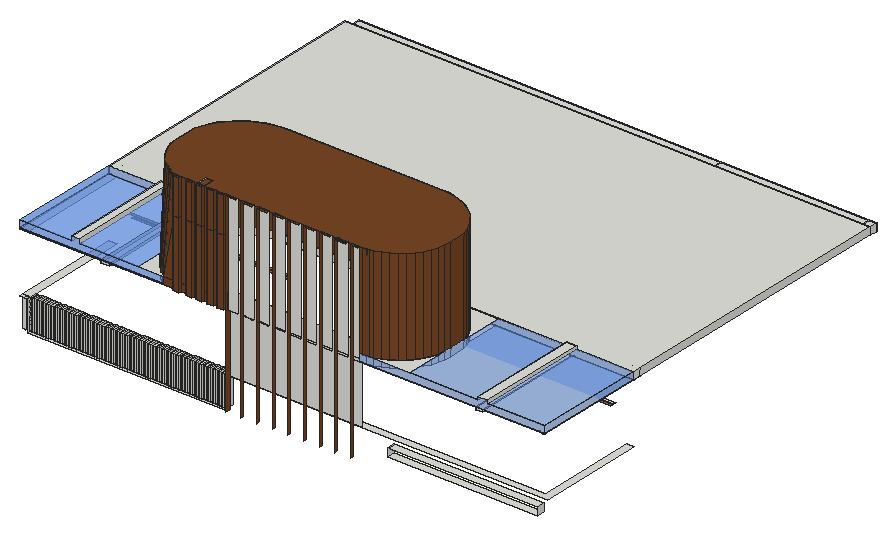
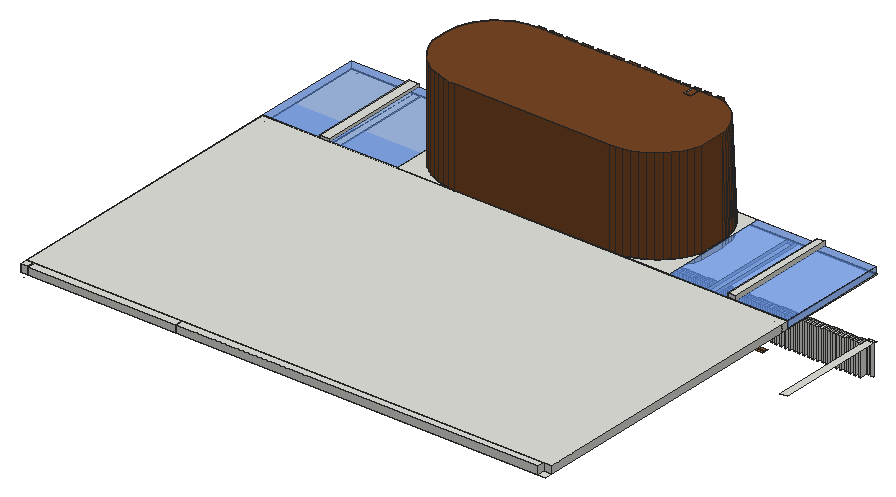
# SketchUp Ruby script. Lengths in inches.
U = 1.inch
M = Sketchup.active_model
def pt(a) = Geom::Point3d.new(a.map { |v| v * U })
def face(e, loops, mat)
  f = e.add_face(loops[0].map { |a| pt(a) })
  loops[1..].each { |l| e.add_face(l.map { |a| pt(a) }).erase! }
  f.material = f.back_material = mat if mat
  f
end
# faces: each face lists its corners as indices into pts; further lists are holes
def faces(e, pts, list, mat = nil) = list.each { |f| face(e, (f[0].is_a?(Array) ? f : [f]).map { |l| l.map { |i| pts[i] } }, mat) }
# xy, xz, yz: faces in a plane at the given z, y or x. An outline is a flat list of corners, or four numbers for a rectangle; further outlines are holes
def ring(l) = l.size == 4 ? [[l[0], l[1]], [l[2], l[1]], [l[2], l[3]], [l[0], l[3]]] : l.each_slice(2).to_a
def flat(e, list, mat, &to3) = list.each { |f| face(e, (f[0].is_a?(Array) ? f : [f]).map { |l| ring(l).map { |u, v| to3.(u, v) } }, mat) }
def xy(e, z, list, mat = nil) = flat(e, list, mat) { |x, y| [x, y, z] }
def xz(e, y, list, mat = nil) = flat(e, list, mat) { |x, z| [x, y, z] }
def yz(e, x, list, mat = nil) = flat(e, list, mat) { |y, z| [x, y, z] }
def lines(e, pts, list) = list.each { |a, b| e.add_line(pt(pts[a]), pt(pts[b])) }
# prism: a flat outline (further loops are holes) pulled along v
def prism(e, loops, v, mat = nil)
  f = face(e, loops, mat); d = Geom::Vector3d.new(v.map { |x| x * U })
  f.pushpull(f.normal.samedirection?(d) ? d.length : -d.length)
end
def box(e, o, s, mat = nil) = prism(e, [[o, [o[0] + s[0], o[1], o[2]], [o[0] + s[0], o[1] + s[1], o[2]], [o[0], o[1] + s[1], o[2]]]], [0, 0, s[2]], mat)
def at(x, y, z, deg = 0) = Geom::Transformation.translation(pt([x, y, z])) * Geom::Transformation.rotation(ORIGIN, Z_AXIS, deg.degrees)
def axes(o, x, y, z) = Geom::Transformation.new([*x, 0, *y, 0, *z, 0, *pt(o).to_a, 1])
def part(name) = M.definitions.add(name)
# library, detail: a bought-in or finely detailed component or shape, given as its bounding box
def library(name, o, s) = part(name).tap { |d| box(d.entities, o, s) }
def detail(e, o, s) = box(e.add_group.entities, o, s)
def put(e, d, t, mat = nil) = e.add_instance(d, t).tap { |i| i.material = mat if mat }
def group(e, t, mat = nil) = e.add_group.tap { |g| g.transformation = t; g.material = mat if mat }.entities
root = M.entities
M.materials.add("[Translucent Glass Blue]").color = [100, 149, 237]
M.materials["[Translucent Glass Blue]"].alpha = 0.5
M.materials.add("[Wood Bamboo]").color = [177, 105, 43]
M.materials.add("[Wood Veneer 01]").color = [120, 70, 37]
xy(root,503.6,[[9.45,3,248.625,6],[9.45,6,11.73,15],[15,6,17.29,15],[20.5625,6,22.86,15],[26.125,6,28.42,15],
  [31.6875,6,33.98,15],[37.25,6,39.54,15],[42.8125,6,45.11,15],[48.375,6,50.67,15],[53.9375,6,56.23,15],
  [59.5,6,61.79,15],[65.0625,6,67.36,15],[70.625,6,72.92,15],[76.1875,6,78.48,15],[81.75,6,84.04,15],
  [87.3125,6,89.61,15],[92.875,6,95.17,15],[98.4375,6,100.73,15],[104,6,106.29,15],[109.5625,6,111.86,15],
  [115.125,6,117.42,15],[120.6875,6,122.98,15],[126.25,6,128.54,15],[131.8125,6,134.11,15],[137.375,6,139.67,15],
  [142.9375,6,145.23,15],[148.5,6,150.79,15],[154.0625,6,156.36,15],[159.625,6,161.92,15],[165.1875,6,167.48,15],
  [170.75,6,173.04,15],[176.3125,6,178.61,15],[181.875,6,184.17,15],[187.4375,6,189.73,15],[193,6,195.29,15],
  [198.5625,6,200.86,15],[204.125,6,206.42,15],[209.6875,6,211.98,15],[215.25,6,217.54,15],[220.8125,6,223.11,15],
  [226.375,6,228.67,15],[231.9375,6,234.23,15],[237.5,6,239.79,15],[243.0625,6,245.36,15]])
xy(root,519.5625,[[439.02,6,618.46,15]])
xy(root,529,[[439.02,6,618.46,15]])
xy(root,540,[[0,3,9.45,6],[0,6,9.45,6,9.45,15,9,15,9,136.3125,0,136.3125],[11.73,6,15,15],[17.29,6,20.5625,15],[22.86,6,26.125,15],
  [28.42,6,31.6875,15],[33.98,6,37.25,15],[39.54,6,42.8125,15],[45.11,6,48.375,15],[50.67,6,53.9375,15],
  [56.23,6,59.5,15],[61.79,6,65.0625,15],[67.36,6,70.625,15],[72.92,6,76.1875,15],[78.48,6,81.75,15],
  [84.04,6,87.3125,15],[89.61,6,92.875,15],[95.17,6,98.4375,15],[100.73,6,104,15],[106.29,6,109.5625,15],
  [111.86,6,115.125,15],[117.42,6,120.6875,15],[122.98,6,126.25,15],[128.54,6,131.8125,15],[134.11,6,137.375,15],
  [139.67,6,142.9375,15],[145.23,6,148.5,15],[150.79,6,154.0625,15],[156.36,6,159.625,15],[161.92,6,165.1875,15],
  [167.48,6,170.75,15],[173.04,6,176.3125,15],[178.61,6,181.875,15],[184.17,6,187.4375,15],[189.73,6,193,15],
  [195.29,6,198.5625,15],[200.86,6,204.125,15],[206.42,6,209.6875,15],[211.98,6,215.25,15],[217.54,6,220.8125,15],
  [223.11,6,226.375,15],[228.67,6,231.9375,15],[234.23,6,237.5,15],[239.79,6,243.0625,15],[245.36,6,630,6,630,136.3125,621,136.3125,621,15,245.36,15]])
xy(root,576.5625,[[29.31,133.3125,65.31,136.3125],[69.34,133.3125,101.31,136.3125],[143.85,133.3125,179.85,136.3125],[182.97,133.3125,215.85,136.3125],[428.86,133.3125,464.86,136.3125],
  [469.18,133.3125,500.86,136.3125],[532.86,133.3125,568.86,136.3125],[572.23,133.3125,604.86,136.3125]],"[Wood Bamboo]")
xy(root,579.5625,[[425.86,133.3125,503.86,136.3125],[529.86,133.3125,607.86,136.3125]])
xy(root,579.5625,[[26.31,133.3125,104.31,136.3125],[140.85,133.3125,218.85,136.3125]],"[Wood Bamboo]")
xy(root,612,[[185.21,0,193.08,3],[200.4,0,208.27,3],[212.61,0,220.48,3],[226.11,0,233.98,3],[238.11,0,245.98,3],
  [0,3,9,136.3125],[0,136.3125,9,145.3125],[9,136.3125,629.5625,145.3125],[629.5625,136.3125,630,136.94],[629.5625,136.94,630,145.3125],
  [0,145.3125,9,490.375],[9,145.3125,621,490.375],[621,145.3125,629.5625,490.375],[629.5625,145.3125,630,490.375],[0,490.375,9,499.375],
  [9,490.375,443.23,499.375],[443.23,490.375,620.5,499.375],[620.5,490.375,620.75,497.0625],[620.75,490.375,621,499.375],[621,490.375,628.8125,499.375],
  [628.8125,490.375,629.5625,499.375],[629.5625,490.375,630,499.375],[620.5,497.0625,620.75,499.3125],[620.5,499.3125,620.75,499.375]])
xy(root,612.0625,[[406.875,3,414.84,3.52,422.66,5.08,430.22,7.64,437.375,11.17,444.01,15.6,450.01,20.87,455.27,26.86,459.7,33.5,463.23,40.65,465.79,48.21,467.35,56.03,467.87,64,467.87,83.88,465.38,91.23,462.12,98.27,458.11,104.91,453.41,111.08,448.07,116.7,442.15,121.72,435.73,126.07,428.87,129.7,421.66,132.57,414.1875,134.64,406.53,135.89,398.79,136.3125,629.5625,136.3125,629.5625,3]])
xy(root,612.75,[[0,3,0,136.3125,213.71,136.3125,205.95,135.9,198.27,134.65,190.78,132.6,183.55,129.75,176.66,126.15,170.2,121.83,164.24,116.84,158.84,111.25,154.08,105.11,149.99,98.5,146.64,91.48,144.06,84.15,144.06,52.64,144.28,47.64,144.93,42.68,146.01,37.8,147.51,33.03,149.43,28.41,151.73,23.98,154.42,19.76,157.46,15.8,160.84,12.11,164.53,8.73,168.49,5.6875,172.71,3]],"[Translucent Glass Blue]")
xy(root,621,[[142.34,3,172.71,3,168.49,5.6875,164.53,8.73,160.84,12.11,157.46,15.8,154.42,19.76,151.73,23.98,149.43,28.41,147.51,33.03,146.01,37.8,144.93,42.68,144.28,47.64,144.06,52.64,144.06,84.15,146.64,91.48,149.99,98.5,154.08,105.11,158.84,111.25,164.24,116.84,170.2,121.83,176.66,126.15,183.55,129.75,190.78,132.6,198.27,134.65,205.95,135.9,213.71,136.3125,142.34,136.3125],[406.875,3,467.9,3,467.9,136.3125,398.79,136.3125,406.53,135.89,414.1875,134.64,421.66,132.57,428.87,129.7,435.73,126.07,442.15,121.72,448.07,116.7,453.41,111.08,458.11,104.91,462.12,98.27,465.38,91.23,467.87,83.88,467.87,64,467.35,56.03,465.79,48.21,463.23,40.65,459.7,33.5,455.27,26.86,450.01,20.87,444.01,15.6,437.375,11.17,430.22,7.64,422.66,5.08,414.84,3.52],[0,136.3125,630,490.375],[9,490.375,443.23,499.375],[443.23,490.375,620.5,499.375],
  [621,490.375,630,499.375]])
xy(root,621,[[0,3,62.18,136.3125],[71.17,3,142.34,136.3125],[467.9,3,548.73,136.3125],[560.78,3,629.5625,136.3125]],"[Translucent Glass Blue]")
xy(root,624.3125,[[548.73,3,560.78,136.3125]])
xy(root,626.25,[[62.18,3,71.17,136.3125]])
xy(root,692.5,[[185.21,0,193.08,3],[200.4,0,208.27,3],[212.61,0,220.48,3],[226.11,0,233.98,3],[238.11,0,245.98,3],
  [212.61,3,220.48,15.6875]])
xy(root,735.21,[[380.31,0,392.78,3]])
xy(root,735.4375,[[185.21,0,193.08,3],[200.4,0,208.27,3],[212.61,0,220.48,3],[226.11,0,233.98,3],[238.11,0,245.98,3],
  [248.625,0,261.1,3],[267.4375,0,279.91,3],[286.25,0,298.72,3],[305.06,0,317.53,3],[323.87,0,336.34,3],
  [342.68,0,355.16,3],[361.49,0,373.97,3],[380.31,0,392.78,3],[399.12,0,406.875,3],[185.21,3,212.61,3,212.61,15.6875,220.48,15.6875,220.48,3,406.875,3,410.86,3.26,414.84,3.52,422.66,5.08,430.22,7.64,437.375,11.17,444.01,15.6,450.01,20.87,455.27,26.86,459.7,33.5,463.23,40.65,465.79,48.21,467.35,56.03,467.87,64,467.87,83.88,465.38,91.23,462.12,98.27,458.11,104.91,453.41,111.08,448.07,116.7,442.15,121.72,435.73,126.07,428.87,129.7,421.66,132.57,414.1875,134.64,406.53,135.89,398.79,136.3125,213.71,136.3125,205.95,135.9,198.27,134.65,190.78,132.6,183.55,129.75,176.66,126.15,170.2,121.83,164.24,116.84,158.84,111.25,154.08,105.11,149.99,98.5,146.64,91.48,144.06,84.15,144.06,52.64,145.24,47.14,146.9,41.76,149.02,36.55,151.59,31.55,154.59,26.79,157.98,22.31,161.76,18.14,165.88,14.3125,170.33,10.86,175.05,7.81,180.03,5.18],
  [212.61,3,220.48,15.6875]],"[Wood Veneer 01]")
xz(root,0,[[185.21,612,193.08,692.5],[200.4,612,208.27,692.5],[212.61,612,220.48,692.5],[226.11,612,233.98,692.5],[238.11,612,245.98,692.5],
  [185.21,692.5,193.08,735.4375],[200.4,692.5,208.27,735.4375],[212.61,692.5,220.48,735.4375],[226.11,692.5,233.98,735.4375],[238.11,692.5,245.98,735.4375],
  [380.31,735.21,392.78,735.4375]],"[Wood Veneer 01]")
xz(root,3,[[546.58,609.5,555.5,609.5,555.5,612,629.5625,612,629.5625,612.0625,406.875,612.0625,406.875,612,546.58,612],[185.21,612,193.08,621],[200.4,612,208.27,621],[212.61,612,220.48,621],[226.11,612,233.98,621],
  [238.11,612,245.98,621],[248.625,612,261.1,735.4375],[267.4375,612,279.91,612.375],[286.25,612,298.72,612.75],[305.06,612,317.53,613.125],
  [323.87,612,336.34,613.5],[342.68,612,355.16,613.875],[361.49,612,373.97,614.25],[380.31,612,392.78,614.625],[399.12,612,406.875,615],
  [267.4375,612.375,279.91,735.4375],[286.25,612.75,298.72,735.4375],[305.06,613.125,317.53,735.4375],[323.87,613.5,336.34,735.4375],[342.68,613.875,355.16,735.4375],
  [361.49,614.25,373.97,735.4375],[380.31,614.625,392.78,735.21],[399.12,615,406.875,735.4375],[185.21,621,193.08,692.5],[200.4,621,208.27,692.5],
  [212.61,621,220.48,692.5],[226.11,621,233.98,692.5],[238.11,621,245.98,692.5],[185.21,692.5,193.08,735.4375],[200.4,692.5,208.27,735.4375],
  [212.61,692.5,220.48,735.4375],[226.11,692.5,233.98,735.4375],[238.11,692.5,245.98,735.4375],[380.31,735.21,392.78,735.4375]])
xz(root,3,[[406.875,612.0625,629.5625,612.0625,629.5625,621,560.78,621,560.78,624.3125,548.73,624.3125,548.73,621,406.875,621],[0,612.75,172.71,612.75,172.71,621,71.17,621,71.17,626.25,62.18,626.25,62.18,621,0,621]],"[Translucent Glass Blue]")
xz(root,3,[[0,612,185.21,612,185.21,621,172.71,621,172.71,612.75,0,612.75],[193.08,612,200.4,621],[208.27,612,212.61,621],[220.48,612,226.11,621],[233.98,612,238.11,621],
  [245.98,612,248.625,621],[172.71,621,185.21,621,185.21,692.5],[193.08,621,200.4,735.4375],[208.27,621,212.61,735.4375],[220.48,621,226.11,735.4375],
  [233.98,621,238.11,735.4375],[245.98,621,248.625,735.4375]],"[Wood Veneer 01]")
xz(root,6,[[0.61,503.6,3.875,540],[6.17,503.6,9.4375,540],[11.73,503.6,15,540],[17.29,503.6,20.5625,540],[22.86,503.6,26.125,540],
  [28.42,503.6,31.6875,540],[33.98,503.6,37.25,540],[39.54,503.6,42.8125,540],[45.11,503.6,48.375,540],[50.67,503.6,53.9375,540],
  [56.23,503.6,59.5,540],[61.79,503.6,65.0625,540],[67.36,503.6,70.625,540],[72.92,503.6,76.1875,540],[78.48,503.6,81.75,540],
  [84.04,503.6,87.3125,540],[89.61,503.6,92.875,540],[95.17,503.6,98.4375,540],[100.73,503.6,104,540],[106.29,503.6,109.5625,540],
  [111.86,503.6,115.125,540],[117.42,503.6,120.6875,540],[122.98,503.6,126.25,540],[128.54,503.6,131.8125,540],[134.11,503.6,137.375,540],
  [139.67,503.6,142.9375,540],[145.23,503.6,148.5,540],[150.79,503.6,154.0625,540],[156.36,503.6,159.625,540],[161.92,503.6,165.1875,540],
  [167.48,503.6,170.75,540],[173.04,503.6,176.3125,540],[178.61,503.6,181.875,540],[184.17,503.6,187.4375,540],[189.73,503.6,193,540],
  [195.29,503.6,198.5625,540],[200.86,503.6,204.125,540],[206.42,503.6,209.6875,540],[211.98,503.6,215.25,540],[217.54,503.6,220.8125,540],
  [223.11,503.6,226.375,540],[228.67,503.6,231.9375,540],[234.23,503.6,237.5,540],[239.79,503.6,243.0625,540],[245.36,503.6,248.625,540],
  [248.625,540,406.875,632.0625]])
xz(root,15.6875,[[212.61,692.5,220.48,735.4375]])
xz(root,136.3125,[[546.58,609.5625,555.5,612.0625],[0,612,0,612.75,213.71,612.75,213.71,621,398.79,621,398.79,612.0625,546.58,612.0625,546.58,612],[546.58,612,555.5,612.0625],[555.5,612,629.5625,612.0625],[629.5625,612,630,621],
  [398.79,612.0625,629.5625,621],[0,612.75,213.71,621],[62.18,621,71.17,626.25],[548.73,621,560.78,624.3125]])
xz(root,136.3125,[[213.71,621,398.79,735.4375]],"[Wood Veneer 01]")
xz(root,490.375,[[0,612,9,621],[9,612,443.23,621],[443.23,612,620.5,621],[620.5,612,620.75,621],[620.75,612,621,621],
  [621,612,630,621]])
xz(root,499.375,[[9,612,443.23,621],[443.23,612,620.5,621],[621,612,630,621]])
yz(root,0,[[3,612,136.3125,612.75],[136.3125,612,145.3125,621],[145.3125,612,490.375,621]])
yz(root,0,[[3,612.75,136.3125,621]],"[Translucent Glass Blue]")
yz(root,9,[[490.375,612,499.375,621]])
yz(root,9.45,[[3,503.6,6,540],[6,503.6,15,540]])
yz(root,11.73,[[6,503.6,15,540]])
yz(root,15,[[6,503.6,15,540]])
yz(root,17.29,[[6,503.6,15,540]])
yz(root,20.5625,[[6,503.6,15,540]])
yz(root,22.86,[[6,503.6,15,540]])
yz(root,26.125,[[6,503.6,15,540]])
yz(root,28.42,[[6,503.6,15,540]])
yz(root,31.6875,[[6,503.6,15,540]])
yz(root,33.98,[[6,503.6,15,540]])
yz(root,37.25,[[6,503.6,15,540]])
yz(root,39.54,[[6,503.6,15,540]])
yz(root,42.8125,[[6,503.6,15,540]])
yz(root,45.11,[[6,503.6,15,540]])
yz(root,48.375,[[6,503.6,15,540]])
yz(root,50.67,[[6,503.6,15,540]])
yz(root,53.9375,[[6,503.6,15,540]])
yz(root,56.23,[[6,503.6,15,540]])
yz(root,59.5,[[6,503.6,15,540]])
yz(root,61.79,[[6,503.6,15,540]])
yz(root,62.18,[[3,621,136.3125,626.25]])
yz(root,65.0625,[[6,503.6,15,540]])
yz(root,67.36,[[6,503.6,15,540]])
yz(root,70.625,[[6,503.6,15,540]])
yz(root,71.17,[[3,621,136.3125,626.25]])
yz(root,72.92,[[6,503.6,15,540]])
yz(root,76.1875,[[6,503.6,15,540]])
yz(root,78.48,[[6,503.6,15,540]])
yz(root,81.75,[[6,503.6,15,540]])
yz(root,84.04,[[6,503.6,15,540]])
yz(root,87.3125,[[6,503.6,15,540]])
yz(root,89.61,[[6,503.6,15,540]])
yz(root,92.875,[[6,503.6,15,540]])
yz(root,95.17,[[6,503.6,15,540]])
yz(root,97.1,[[3.02,608.875,3,612,136.3125,612.75,136.33,609.625]])
yz(root,98.4375,[[6,503.6,15,540]])
yz(root,100.73,[[6,503.6,15,540]])
yz(root,104,[[6,503.6,15,540]])
yz(root,106.29,[[6,503.6,15,540]])
yz(root,106.85,[[3.02,608.875,136.33,609.625,136.3125,612.75,3,612]])
yz(root,109.5625,[[6,503.6,15,540]])
yz(root,111.86,[[6,503.6,15,540]])
yz(root,115.125,[[6,503.6,15,540]])
yz(root,117.42,[[6,503.6,15,540]])
yz(root,120.6875,[[6,503.6,15,540]])
yz(root,122.98,[[6,503.6,15,540]])
yz(root,126.25,[[6,503.6,15,540]])
yz(root,128.54,[[6,503.6,15,540]])
yz(root,131.8125,[[6,503.6,15,540]])
yz(root,134.11,[[6,503.6,15,540]])
yz(root,137.375,[[6,503.6,15,540]])
yz(root,139.67,[[6,503.6,15,540]])
yz(root,142.9375,[[6,503.6,15,540]])
yz(root,144.06,[[52.64,612.75,84.15,621]])
yz(root,144.06,[[52.64,621,84.15,735.4375]],"[Wood Veneer 01]")
yz(root,145.23,[[6,503.6,15,540]])
yz(root,148.5,[[6,503.6,15,540]])
yz(root,150.79,[[6,503.6,15,540]])
yz(root,154.0625,[[6,503.6,15,540]])
yz(root,156.36,[[6,503.6,15,540]])
yz(root,159.625,[[6,503.6,15,540]])
yz(root,161.92,[[6,503.6,15,540]])
yz(root,165.1875,[[6,503.6,15,540]])
yz(root,167.48,[[6,503.6,15,540]])
yz(root,170.75,[[6,503.6,15,540]])
yz(root,173.04,[[6,503.6,15,540]])
yz(root,176.3125,[[6,503.6,15,540]])
yz(root,178.61,[[6,503.6,15,540]])
yz(root,181.875,[[6,503.6,15,540]])
yz(root,184.17,[[6,503.6,15,540]])
yz(root,185.21,[[0,612,3,692.5],[0,692.5,3,735.4375]],"[Wood Veneer 01]")
yz(root,187.4375,[[6,503.6,15,540]])
yz(root,189.73,[[6,503.6,15,540]])
yz(root,193,[[6,503.6,15,540]])
yz(root,193.08,[[0,612,3,692.5],[0,692.5,3,735.4375]],"[Wood Veneer 01]")
yz(root,195.29,[[6,503.6,15,540]])
yz(root,198.5625,[[6,503.6,15,540]])
yz(root,200.4,[[0,612,3,692.5],[0,692.5,3,735.4375]],"[Wood Veneer 01]")
yz(root,200.86,[[6,503.6,15,540]])
yz(root,204.125,[[6,503.6,15,540]])
yz(root,206.42,[[6,503.6,15,540]])
yz(root,208.27,[[0,612,3,692.5],[0,692.5,3,735.4375]],"[Wood Veneer 01]")
yz(root,209.6875,[[6,503.6,15,540]])
yz(root,211.98,[[6,503.6,15,540]])
yz(root,212.61,[[3,692.5,15.6875,735.4375]])
yz(root,212.61,[[0,612,3,692.5],[0,692.5,3,735.4375]],"[Wood Veneer 01]")
yz(root,215.25,[[6,503.6,15,540]])
yz(root,217.54,[[6,503.6,15,540]])
yz(root,220.48,[[3,692.5,15.6875,735.4375]])
yz(root,220.48,[[0,612,3,692.5],[0,692.5,3,735.4375]],"[Wood Veneer 01]")
yz(root,220.8125,[[6,503.6,15,540]])
yz(root,223.11,[[6,503.6,15,540]])
yz(root,226.11,[[0,612,3,692.5],[0,692.5,3,735.4375]],"[Wood Veneer 01]")
yz(root,226.375,[[6,503.6,15,540]])
yz(root,228.67,[[6,503.6,15,540]])
yz(root,231.9375,[[6,503.6,15,540]])
yz(root,233.98,[[0,612,3,692.5],[0,692.5,3,735.4375]],"[Wood Veneer 01]")
yz(root,234.23,[[6,503.6,15,540]])
yz(root,237.5,[[6,503.6,15,540]])
yz(root,238.11,[[0,612,3,692.5],[0,692.5,3,735.4375]],"[Wood Veneer 01]")
yz(root,239.79,[[6,503.6,15,540]])
yz(root,243.0625,[[6,503.6,15,540]])
yz(root,245.36,[[6,503.6,15,540]])
yz(root,245.98,[[0,612,3,692.5],[0,692.5,3,735.4375]],"[Wood Veneer 01]")
yz(root,248.625,[[0,503.6,0,612,3,612,3,632.0625,6,632.0625,6,503.6],[0,612,3,735.4375]],"[Wood Veneer 01]")
yz(root,267.4375,[[0,503.98,3,735.4375]],"[Wood Veneer 01]")
yz(root,286.25,[[0,504.35,3,612],[0,612,3,735.4375]],"[Wood Veneer 01]")
yz(root,305.06,[[0,504.73,3,735.4375]],"[Wood Veneer 01]")
yz(root,323.87,[[0,505.1,3,735.4375]],"[Wood Veneer 01]")
yz(root,342.68,[[0,505.48,3,735.4375]],"[Wood Veneer 01]")
yz(root,361.49,[[0,505.85,3,735.4375]],"[Wood Veneer 01]")
yz(root,380.31,[[0,506.23,3,735.21],[0,735.21,3,735.4375]],"[Wood Veneer 01]")
yz(root,392.78,[[0,735.21,3,735.4375]],"[Wood Veneer 01]")
yz(root,399.12,[[0,506.6,3,735.4375]],"[Wood Veneer 01]")
yz(root,439.02,[[6,519.5625,15,529]])
yz(root,443.23,[[490.375,612,499.375,621]])
yz(root,467.87,[[64,612.0625,83.88,621]])
yz(root,467.87,[[64,621,83.88,735.4375]],"[Wood Veneer 01]")
yz(root,546.58,[[3,609.5,3,612,136.3125,612.0625,136.3125,609.5625]])
yz(root,548.73,[[3,621,136.3125,624.3125]])
yz(root,555.5,[[3,609.5,136.3125,609.5625,136.3125,612.0625,3,612]])
yz(root,560.78,[[3,621,136.3125,624.3125]])
yz(root,618.46,[[6,519.5625,15,529]])
yz(root,620.5,[[490.375,612,499.375,621]])
yz(root,621,[[490.375,612,499.375,621]])
yz(root,629.5625,[[3,612,136.3125,612,136.3125,612.0625],[3,612,136.3125,612.0625,3,612.0625]])
yz(root,629.5625,[[3,612.0625,136.3125,621]],"[Translucent Glass Blue]")
yz(root,630,[[136.3125,612,145.3125,621],[145.3125,612,490.375,621],[490.375,612,499.375,621]])
p = [[106.85,136.33,609.625],[106.85,3.02,608.875],[97.1,3.02,608.875],[97.1,136.33,609.625],[106.85,3,612],[97.1,3,612],
  [546.58,136.3125,609.5625],[555.5,136.3125,609.5625],[555.5,3,609.5],[546.58,3,609.5],[97.1,136.3125,612.75],[106.85,136.3125,612.75],
  [463.59,136.3125,612.0625],[546.58,136.3125,612.0625],[546.58,3,612],[463.59,3,612],[629.5625,3,612],[555.5,3,612],
  [555.5,136.3125,612.0625],[629.5625,136.3125,612.0625],[406.875,3,621],[414.84,3.52,621],[414.84,3.52,612.0625],[406.875,3,612.0625],
  [406.875,3,615],[422.66,5.08,621],[422.66,5.08,612.0625],[430.22,7.64,621],[430.22,7.64,612.0625],[437.375,11.17,621],
  [437.375,11.17,612.0625],[444.01,15.6,621],[444.01,15.6,612.0625],[450.01,20.87,621],[450.01,20.87,612.0625],[455.27,26.86,621],
  [455.27,26.86,612.0625],[459.7,33.5,621],[459.7,33.5,612.0625],[463.23,40.65,621],[463.23,40.65,612.0625],[465.79,48.21,621],
  [465.79,48.21,612.0625],[467.35,56.03,621],[467.35,56.03,612.0625],[467.87,64,621],[467.87,64,612.0625],[467.87,83.88,621],
  [465.38,91.23,621],[465.38,91.23,612.0625],[467.87,83.88,612.0625],[462.12,98.27,621],[462.12,98.27,612.0625],[458.11,104.91,621],
  [458.11,104.91,612.0625],[453.41,111.08,621],[453.41,111.08,612.0625],[448.07,116.7,621],[448.07,116.7,612.0625],[442.15,121.72,621],
  [442.15,121.72,612.0625],[435.73,126.07,621],[435.73,126.07,612.0625],[428.87,129.7,621],[428.87,129.7,612.0625],[421.66,132.57,621],
  [421.66,132.57,612.0625],[414.1875,134.64,621],[414.1875,134.64,612.0625],[406.53,135.89,621],[406.53,135.89,612.0625],[398.79,136.3125,621],
  [398.79,136.3125,612.0625],[168.49,5.6875,621],[172.71,3,621],[172.71,3,612.75],[168.49,5.6875,612.75],[164.53,8.73,621],
  [164.53,8.73,612.75],[160.84,12.11,621],[160.84,12.11,612.75],[157.46,15.8,621],[157.46,15.8,612.75],[154.42,19.76,621],
  [154.42,19.76,612.75],[151.73,23.98,621],[151.73,23.98,612.75],[149.43,28.41,621],[149.43,28.41,612.75],[147.51,33.03,621],
  [147.51,33.03,612.75],[146.01,37.8,621],[146.01,37.8,612.75],[144.93,42.68,621],[144.93,42.68,612.75],[144.28,47.64,621],
  [144.28,47.64,612.75],[144.06,52.64,621],[144.06,52.64,612.75],[146.64,91.48,621],[144.06,84.15,621],[144.06,84.15,612.75],
  [146.64,91.48,612.75],[149.99,98.5,621],[149.99,98.5,612.75],[154.08,105.11,621],[154.08,105.11,612.75],[158.84,111.25,621],
  [158.84,111.25,612.75],[164.24,116.84,621],[164.24,116.84,612.75],[170.2,121.83,621],[170.2,121.83,612.75],[176.66,126.15,621],
  [176.66,126.15,612.75],[183.55,129.75,621],[183.55,129.75,612.75],[190.78,132.6,621],[190.78,132.6,612.75],[198.27,134.65,621],
  [198.27,134.65,612.75],[205.95,135.9,621],[205.95,135.9,612.75],[213.71,136.3125,621],[213.71,136.3125,612.75],[180.03,5.18,735.4375],
  [185.21,3,692.5],[414.84,3.52,735.4375],[410.86,3.26,735.4375],[406.875,3,735.4375],[406.875,3,632.0625],[410.87,3.07,621],
  [417.83,3.52,621],[417.82,3.72,735.4375],[422.66,5.08,735.4375],[430.22,7.64,735.4375],[175.05,7.81,735.4375],[437.375,11.17,735.4375],
  [170.33,10.86,735.4375],[165.88,14.3125,735.4375],[444.01,15.6,735.4375],[161.76,18.14,735.4375],[450.01,20.87,735.4375],[157.98,22.31,735.4375],
  [455.27,26.86,735.4375],[154.59,26.79,735.4375],[151.59,31.55,735.4375],[459.7,33.5,735.4375],[149.02,36.55,735.4375],[463.23,40.65,735.4375],
  [146.9,41.76,735.4375],[465.79,48.21,735.4375],[145.24,47.14,735.4375],[144.06,52.64,735.4375],[467.35,56.03,735.4375],[467.87,64,735.4375],
  [465.38,91.23,735.4375],[467.87,83.88,735.4375],[144.06,84.15,735.4375],[146.64,91.48,735.4375],[462.12,98.27,735.4375],[149.99,98.5,735.4375],
  [458.11,104.91,735.4375],[154.08,105.11,735.4375],[453.41,111.08,735.4375],[158.84,111.25,735.4375],[448.07,116.7,735.4375],[164.24,116.84,735.4375],
  [442.15,121.72,735.4375],[170.2,121.83,735.4375],[435.73,126.07,735.4375],[176.66,126.15,735.4375],[183.55,129.75,735.4375],[428.87,129.7,735.4375],
  [190.78,132.6,735.4375],[421.66,132.57,735.4375],[198.27,134.65,735.4375],[414.1875,134.64,735.4375],[406.53,135.89,735.4375],[205.95,135.9,735.4375],
  [213.71,136.3125,735.4375],[398.79,136.3125,735.4375],[185.21,3,735.4375],[621,6,612],[620.75,6,612],[620.75,506,612],
  [620.5,506,612],[9,145.3125,612],[9,145.3125,621],[621,145.3125,612],[621,145.3125,621]]
faces(root,p,[[0,1,2,3],[4,5,2,1],[6,7,8,9],[10,11,0,3],[20,21,22,23,24],[21,25,26,22],[25,27,28,26],[27,29,30,28],
  [29,31,32,30],[31,33,34,32],[33,35,36,34],[35,37,38,36],[37,39,40,38],[39,41,42,40],[41,43,44,42],[43,45,46,44],
  [47,48,49,50],[48,51,52,49],[51,53,54,52],[53,55,56,54],[55,57,58,56],[57,59,60,58],[59,61,62,60],[61,63,64,62],
  [63,65,66,64],[65,67,68,66],[67,69,70,68],[69,71,72,70],[73,74,75,76],[77,73,76,78],[79,77,78,80],[81,79,80,82],
  [83,81,82,84],[85,83,84,86],[87,85,86,88],[89,87,88,90],[91,89,90,92],[93,91,92,94],[95,93,94,96],[97,95,96,98],
  [99,100,101,102],[103,99,102,104],[105,103,104,106],[107,105,106,108],[109,107,108,110],[111,109,110,112],[113,111,112,114],[115,113,114,116],
  [117,115,116,118],[119,117,118,120],[121,119,120,122],[123,121,122,124]])
faces(root,p,[[12,13,14,15],[16,17,18,19]],"[Translucent Glass Blue]")
faces(root,p,[[125,73,126],[74,126,73],[20,21,127,128,129,130],[128,131,132,133,127],[21,25,134,127],[25,27,135,134],[73,125,77],[136,77,125],
  [27,29,137,135],[77,136,79],[138,79,136],[138,139,79],[29,31,140,137],[81,79,139],[139,141,81],[31,33,142,140],
  [83,81,141],[141,143,83],[85,83,143],[33,35,144,142],[143,145,85],[87,85,145],[145,146,87],[35,37,147,144],
  [89,87,146],[146,148,89],[91,89,148],[37,39,149,147],[148,150,91],[93,91,150],[39,41,151,149],[150,152,93],
  [95,93,152],[152,153,95],[97,95,153],[41,43,154,151],[43,45,155,154],[47,48,156,157],[99,100,158,159],[48,51,160,156],
  [103,99,159,161],[51,53,162,160],[105,103,161,163],[53,55,164,162],[107,105,163,165],[55,57,166,164],[109,107,165,167],[57,59,168,166],
  [111,109,167,169],[59,61,170,168],[113,111,169,171],[115,113,171,172],[61,63,173,170],[117,115,172,174],[63,65,175,173],[119,117,174,176],
  [65,67,177,175],[67,69,178,177],[121,119,176,179],[123,121,179,180],[69,71,181,178],[182,125,126]],"[Wood Veneer 01]")
lines(root,p,[[183,184],[185,186],[187,188],[189,190]])
